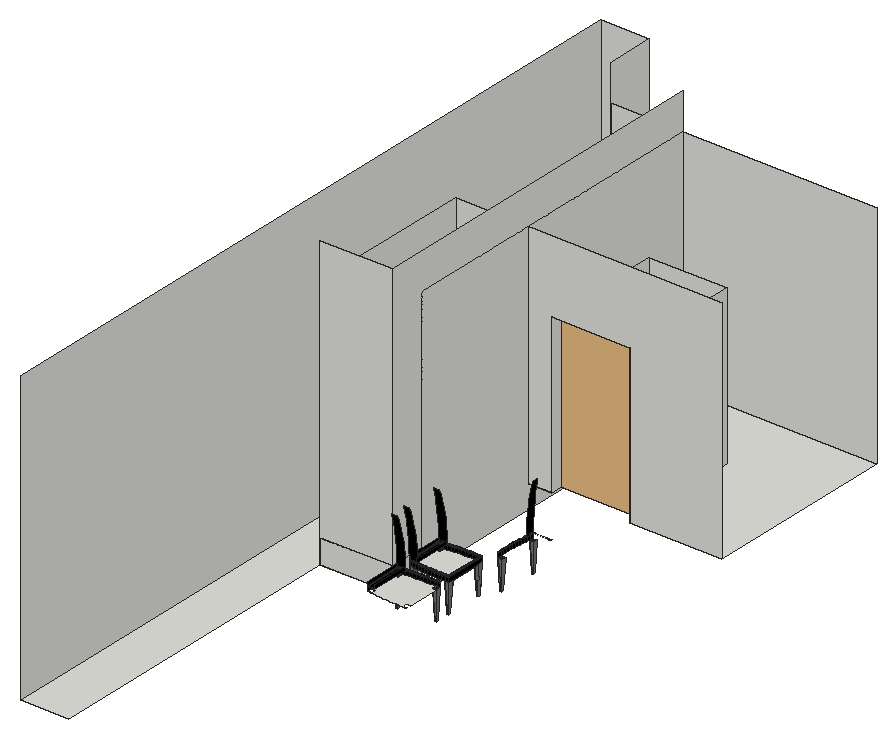
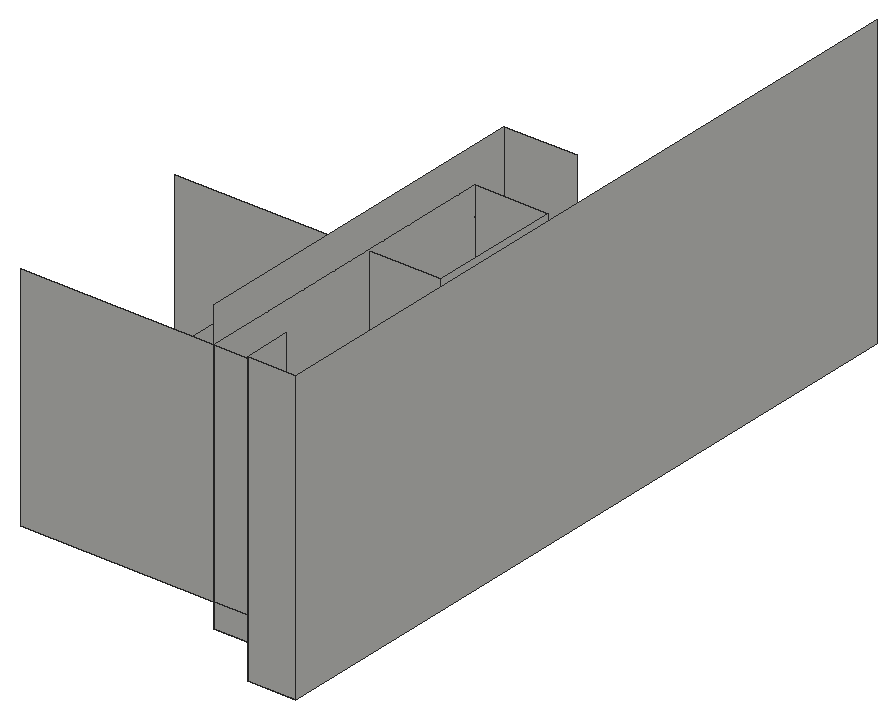
# SketchUp Ruby script. Lengths in inches.
U = 1.inch
M = Sketchup.active_model
def pt(a) = Geom::Point3d.new(a.map { |v| v * U })
def face(e, loops, mat)
  f = e.add_face(loops[0].map { |a| pt(a) })
  loops[1..].each { |l| e.add_face(l.map { |a| pt(a) }).erase! }
  f.material = f.back_material = mat if mat
  f
end
# faces: each face lists its corners as indices into pts; further lists are holes
def faces(e, pts, list, mat = nil) = list.each { |f| face(e, (f[0].is_a?(Array) ? f : [f]).map { |l| l.map { |i| pts[i] } }, mat) }
# xy, xz, yz: faces in a plane at the given z, y or x. An outline is a flat list of corners, or four numbers for a rectangle; further outlines are holes
def ring(l) = l.size == 4 ? [[l[0], l[1]], [l[2], l[1]], [l[2], l[3]], [l[0], l[3]]] : l.each_slice(2).to_a
def flat(e, list, mat, &to3) = list.each { |f| face(e, (f[0].is_a?(Array) ? f : [f]).map { |l| ring(l).map { |u, v| to3.(u, v) } }, mat) }
def xy(e, z, list, mat = nil) = flat(e, list, mat) { |x, y| [x, y, z] }
def xz(e, y, list, mat = nil) = flat(e, list, mat) { |x, z| [x, y, z] }
def yz(e, x, list, mat = nil) = flat(e, list, mat) { |y, z| [x, y, z] }
def lines(e, pts, list) = list.each { |a, b| e.add_line(pt(pts[a]), pt(pts[b])) }
# prism: a flat outline (further loops are holes) pulled along v
def prism(e, loops, v, mat = nil)
  f = face(e, loops, mat); d = Geom::Vector3d.new(v.map { |x| x * U })
  f.pushpull(f.normal.samedirection?(d) ? d.length : -d.length)
end
def box(e, o, s, mat = nil) = prism(e, [[o, [o[0] + s[0], o[1], o[2]], [o[0] + s[0], o[1] + s[1], o[2]], [o[0], o[1] + s[1], o[2]]]], [0, 0, s[2]], mat)
def at(x, y, z, deg = 0) = Geom::Transformation.translation(pt([x, y, z])) * Geom::Transformation.rotation(ORIGIN, Z_AXIS, deg.degrees)
def axes(o, x, y, z) = Geom::Transformation.new([*x, 0, *y, 0, *z, 0, *pt(o).to_a, 1])
def part(name) = M.definitions.add(name)
# library, detail: a bought-in or finely detailed component or shape, given as its bounding box
def library(name, o, s) = part(name).tap { |d| box(d.entities, o, s) }
def detail(e, o, s) = box(e.add_group.entities, o, s)
def put(e, d, t, mat = nil) = e.add_instance(d, t).tap { |i| i.material = mat if mat }
def group(e, t, mat = nil) = e.add_group.tap { |g| g.transformation = t; g.material = mat if mat }.entities
root = M.entities
M.materials.add("Color_008").color = [30, 30, 30]
M.materials.add("[Color M09]").color = [0, 0, 0]
M.materials.add("[Metal Seamed]").color = [118, 119, 115]
c1 = library("Group5\#2",[-22.22,-6.35,0],[42.52,9.29,84.25])
xy(root,0,[[0,0,24,360],[24,156,60,336]])
xy(root,12,[[24,156,60,174],[24,240,72,240,72,300,110.625,300,110.625,240,156,240,156,336,24,336]])
xy(root,12,[[81.769,130.997,82.586,131.814],[100.046,132.018,100.863,132.835],[100.046,139.647,100.863,140.464],[81.769,140.669,82.586,141.485],[81.769,156.903,82.586,157.72],
  [100.046,157.924,100.863,158.741],[104.815,166.733,105.632,167.55],[105.836,185.01,106.653,185.827]],"Color_008")
xy(root,26.704,[[96.409,112.95,94.702,112.965,92.996,113.008,91.291,113.079,89.587,113.178,87.885,113.306,86.185,113.462,84.488,113.646,82.795,113.858,81.105,114.098,83.25,114.098,83.25,116.244,81.105,116.244,81.105,130.333,83.25,130.333,83.25,132.478,81.105,132.478,82.795,132.718,84.488,132.931,86.185,133.115,87.885,133.271,89.587,133.398,91.291,133.498,92.996,133.569,94.702,133.612,96.409,133.626,98.115,133.612,99.822,133.57,101.527,133.499,99.382,133.499,99.382,131.354,101.527,131.354,101.527,115.223,99.382,115.223,99.382,113.077,101.527,113.077,99.822,113.007,98.115,112.964],[96.409,138.856,94.702,138.871,92.996,138.913,91.291,138.984,89.587,139.084,87.885,139.212,86.185,139.367,84.488,139.552,82.795,139.764,81.105,140.004,83.25,140.004,83.25,142.15,81.105,142.15,81.105,156.239,83.25,156.239,83.25,158.384,81.105,158.384,82.795,158.624,84.488,158.837,86.185,159.021,87.885,159.177,89.587,159.304,91.291,159.404,92.996,159.475,94.702,159.517,96.409,159.532,98.115,159.518,99.822,159.476,101.527,159.405,99.382,159.405,99.382,157.26,101.527,157.26,101.527,141.129,99.382,141.129,99.382,138.983,101.527,138.983,99.822,138.913,98.115,138.87]])
xy(root,26.704,[[81.105,130.333,83.25,132.478],[99.382,131.354,101.527,133.499],[99.382,138.983,101.527,141.129],[81.105,140.004,83.25,142.15],[81.105,156.239,83.25,158.384],
  [99.382,157.26,101.527,159.405],[104.151,166.069,106.296,168.214],[105.172,184.346,107.317,186.491]],"Color_008")
xy(root,28.845,[[81.105,114.098,84.642,132.478],[81.105,140.004,84.642,158.384]],"[Color M09]")
xz(root,132.478,[[81.105,28.845,84.642,28.845,84.773,30.816,84.825,32.79,84.797,34.764,84.689,36.736,84.502,38.701,84.235,40.658,83.89,42.602,83.466,44.53,82.965,46.44,82.387,48.328,81.733,50.191,81.004,52.027,78.554,52.027,78.952,50.121,79.316,48.208,79.647,46.29,79.945,44.365,80.208,42.436,80.438,40.503,80.634,38.566,80.797,36.626,80.925,34.683,81.019,32.738,81.079,30.792]],"[Color M09]")
xz(root,140.004,[[81.105,28.845,81.079,30.792,81.019,32.738,80.925,34.683,80.797,36.626,80.634,38.566,80.438,40.503,80.208,42.436,79.945,44.365,79.647,46.29,79.316,48.208,78.952,50.121,78.554,52.027,81.004,52.027,81.733,50.191,82.387,48.328,82.965,46.44,83.466,44.53,83.89,42.602,84.235,40.658,84.502,38.701,84.689,36.736,84.797,34.764,84.825,32.79,84.773,30.816,84.642,28.845]],"[Color M09]")
xz(root,156,[[24,0,60,12],[24,12,60,144]])
xz(root,158.384,[[81.105,28.845,84.642,28.845,84.773,30.816,84.825,32.79,84.797,34.764,84.689,36.736,84.502,38.701,84.235,40.658,83.89,42.602,83.466,44.53,82.965,46.44,82.387,48.328,81.733,50.191,81.004,52.027,78.554,52.027,78.952,50.121,79.316,48.208,79.647,46.29,79.945,44.365,80.208,42.436,80.438,40.503,80.634,38.566,80.797,36.626,80.925,34.683,81.019,32.738,81.079,30.792]],"[Color M09]")
xz(root,174,[[24,12,60,126]])
xz(root,240,[[24,12,72,12,72,90,110.625,90,110.625,12,156,12,156,126,24,126]])
xz(root,300,[[72,12,110.625,90]])
xz(root,336,[[24,0,60,12],[24,12,60,126],[60,12,156,126]])
xz(root,360,[[0,0,24,144]])
yz(root,0,[[0,0,360,144]])
yz(root,24,[[156,0,336,12],[336,0,360,144],[174,12,240,126]])
yz(root,60,[[156,0,336,0,336,126,174,126,174,12,156,12],[156,12,174,12,174,126,336,126,336,144,156,144]])
yz(root,72,[[240,12,300,90]])
yz(root,81.105,[[114.098,26.704,132.478,28.845],[140.004,26.704,158.384,28.845]],"[Color M09]")
yz(root,101.527,[[138.983,26.704,159.405,28.845]],"[Color M09]")
yz(root,105.172,[[182.954,28.845,186.491,28.845,186.517,30.792,186.577,32.738,186.671,34.683,186.799,36.626,186.962,38.566,187.158,40.503,187.388,42.436,187.651,44.365,187.949,46.29,188.28,48.208,188.644,50.121,189.042,52.027,186.592,52.027,185.863,50.191,185.209,48.328,184.631,46.44,184.13,44.53,183.706,42.602,183.361,40.658,183.094,38.701,182.907,36.736,182.799,34.764,182.771,32.79,182.823,30.816]],"[Color M09]")
yz(root,110.625,[[240,12,300,90]])
p = [[82.586,130.997,12],[83.25,130.333,26.704],[81.105,130.333,26.704],[81.769,130.997,12],[81.105,132.478,26.704],[81.769,131.814,12],
  [82.586,131.814,12],[83.25,132.478,26.704],[100.863,132.018,12],[101.527,131.354,26.704],[99.382,131.354,26.704],[100.046,132.018,12],
  [99.382,133.499,26.704],[100.046,132.835,12],[100.863,132.835,12],[101.527,133.499,26.704],[100.863,139.647,12],[101.527,138.983,26.704],
  [99.382,138.983,26.704],[100.046,139.647,12],[99.382,141.129,26.704],[100.046,140.464,12],[100.863,140.464,12],[101.527,141.129,26.704],
  [82.586,140.669,12],[83.25,140.004,26.704],[81.105,140.004,26.704],[81.769,140.669,12],[81.105,142.15,26.704],[81.769,141.485,12],
  [82.586,141.485,12],[83.25,142.15,26.704],[82.586,156.903,12],[83.25,156.239,26.704],[81.105,156.239,26.704],[81.769,156.903,12],
  [81.105,158.384,26.704],[81.769,157.72,12],[82.586,157.72,12],[83.25,158.384,26.704],[100.863,157.924,12],[101.527,157.26,26.704],
  [99.382,157.26,26.704],[100.046,157.924,12],[99.382,159.405,26.704],[100.046,158.741,12],[100.863,158.741,12],[101.527,159.405,26.704],
  [105.632,166.733,12],[106.296,166.069,26.704],[104.151,166.069,26.704],[104.815,166.733,12],[104.151,168.214,26.704],[104.815,167.55,12],
  [105.632,167.55,12],[106.296,168.214,26.704],[106.653,185.01,12],[107.317,184.346,26.704],[105.172,184.346,26.704],[105.836,185.01,12],
  [105.172,186.491,26.704],[105.836,185.827,12],[106.653,185.827,12],[107.317,186.491,26.704],[82.795,132.718,28.845],[82.795,132.718,26.704],
  [81.105,132.478,28.845],[84.488,132.931,28.845],[84.488,132.931,26.704],[86.185,133.115,28.845],[86.185,133.115,26.704],[87.885,133.271,28.845],
  [87.885,133.271,26.704],[89.587,133.398,28.845],[89.587,133.398,26.704],[91.291,133.498,28.845],[91.291,133.498,26.704],[92.996,133.569,28.845],
  [92.996,133.569,26.704],[99.822,133.57,28.845],[99.822,133.57,26.704],[101.527,133.499,28.845],[94.702,133.612,26.704],[94.702,133.612,28.845],
  [96.409,133.626,26.704],[96.409,133.626,28.845],[98.115,133.612,26.704],[98.115,133.612,28.845],[92.996,138.913,26.704],[92.996,138.913,28.845],
  [91.291,138.984,28.845],[91.291,138.984,26.704],[94.702,138.871,28.845],[94.702,138.871,26.704],[96.409,138.856,28.845],[96.409,138.856,26.704],
  [98.115,138.87,28.845],[98.115,138.87,26.704],[99.822,138.913,28.845],[99.822,138.913,26.704],[101.527,138.983,28.845],[89.587,139.084,28.845],
  [89.587,139.084,26.704],[87.885,139.212,28.845],[87.885,139.212,26.704],[86.185,139.367,28.845],[86.185,139.367,26.704],[84.488,139.552,28.845],
  [84.488,139.552,26.704],[82.795,139.764,28.845],[82.795,139.764,26.704],[81.105,140.004,28.845],[82.795,158.624,28.845],[82.795,158.624,26.704],
  [81.105,158.384,28.845],[84.488,158.837,28.845],[84.488,158.837,26.704],[86.185,159.021,28.845],[86.185,159.021,26.704],[87.885,159.177,28.845],
  [87.885,159.177,26.704],[89.587,159.304,28.845],[89.587,159.304,26.704],[91.291,159.404,28.845],[91.291,159.404,26.704],[92.996,159.475,28.845],
  [92.996,159.475,26.704],[99.822,159.476,28.845],[99.822,159.476,26.704],[101.527,159.405,28.845],[94.702,159.517,26.704],[94.702,159.517,28.845],
  [96.409,159.532,26.704],[96.409,159.532,28.845],[98.115,159.518,26.704],[98.115,159.518,28.845],[104.08,167.774,26.704],[104.08,167.774,28.845],
  [104.151,166.069,28.845],[104.038,169.481,26.704],[104.038,169.481,28.845],[104.024,171.1875,26.704],[104.024,171.1875,28.845],[104.038,172.894,26.704],
  [104.038,172.894,28.845],[104.081,174.6,26.704],[104.081,174.6,28.845],[104.152,176.305,28.845],[104.152,176.305,26.704],[104.252,178.009,28.845],
  [104.252,178.009,26.704],[104.379,179.711,28.845],[104.379,179.711,26.704],[104.535,181.411,28.845],[104.535,181.411,26.704],[104.719,183.108,28.845],
  [104.719,183.108,26.704],[104.932,184.801,28.845],[104.932,184.801,26.704],[105.172,186.491,28.845],[81.079,132.478,30.792],[81.079,114.098,30.792],
  [81.105,114.098,28.845],[81.115,132.47,28.992],[81.115,114.107,28.992],[84.773,132.478,30.816],[84.642,132.478,28.845],[84.642,114.098,28.845],
  [84.773,114.098,30.816],[82.796,132.709,28.992],[84.489,132.921,28.992],[86.186,133.105,28.992],[87.886,133.261,28.992],[89.587,133.389,28.992],
  [91.291,133.488,28.992],[92.996,133.559,28.992],[99.821,133.56,28.992],[101.517,133.49,28.992],[94.702,133.602,28.992],[96.409,133.616,28.992],
  [98.115,133.602,28.992],[92.996,138.923,28.992],[91.291,138.994,28.992],[94.702,138.88,28.992],[96.409,138.866,28.992],[98.115,138.88,28.992],
  [99.821,138.922,28.992],[101.517,138.992,28.992],[89.587,139.093,28.992],[101.517,159.396,28.992],[87.886,139.221,28.992],[86.186,139.377,28.992],
  [84.489,139.561,28.992],[82.796,139.773,28.992],[81.115,140.013,28.992],[81.079,158.384,30.792],[81.079,140.004,30.792],[81.115,158.376,28.992],
  [84.773,158.384,30.816],[84.642,158.384,28.845],[84.642,140.004,28.845],[84.773,140.004,30.816],[82.796,158.615,28.992],[84.489,158.827,28.992],
  [86.186,159.011,28.992],[87.886,159.167,28.992],[89.587,159.295,28.992],[91.291,159.394,28.992],[92.996,159.465,28.992],[99.821,159.466,28.992],
  [94.702,159.508,28.992],[96.409,159.522,28.992],[98.115,159.508,28.992],[104.09,167.775,28.992],[104.16,166.079,28.992],[104.048,169.481,28.992],
  [104.034,171.1875,28.992],[104.048,172.894,28.992],[104.091,174.6,28.992],[104.162,176.305,28.992],[104.261,178.009,28.992],[104.389,179.71,28.992],
  [104.545,181.41,28.992],[104.729,183.107,28.992],[104.941,184.8,28.992],[105.18,186.481,28.992],[81.143,132.445,29.137],[81.143,114.132,29.137],
  [81.143,123.288,29.137],[82.8,132.68,29.137],[84.493,132.893,29.137],[86.189,133.077,29.137],[87.888,133.233,29.137],[89.589,133.36,29.137],
  [91.292,133.46,29.137],[92.997,133.531,29.137],[94.703,133.573,29.137],[98.115,133.574,29.137],[99.82,133.531,29.137],[101.489,133.462,29.137],
  [96.409,133.588,29.137],[92.997,138.952,29.137],[91.292,139.023,29.137],[94.703,138.909,29.137],[96.409,138.895,29.137],[98.115,138.909,29.137],
  [99.82,138.951,29.137],[101.489,139.02,29.137],[89.589,139.122,29.137],[101.489,159.368,29.137],[87.888,139.25,29.137],[86.189,139.406,29.137],
  [84.493,139.59,29.137],[82.8,139.802,29.137],[81.143,140.038,29.137],[81.143,158.351,29.137],[81.143,149.194,29.137],[82.8,158.586,29.137],
  [84.493,158.798,29.137],[86.189,158.983,29.137],[87.888,159.138,29.137],[89.589,159.266,29.137],[91.292,159.365,29.137],[92.997,159.436,29.137],
  [94.703,159.479,29.137],[98.115,159.48,29.137],[99.82,159.437,29.137],[96.409,159.494,29.137],[104.119,167.776,29.137],[104.188,166.107,29.137],
  [104.076,169.481,29.137],[104.0625,171.1875,29.137],[104.077,172.893,29.137],[104.119,174.599,29.137],[104.191,176.304,29.137],[104.29,178.007,29.137],
  [104.417,179.708,29.137],[104.573,181.407,29.137],[104.757,183.103,29.137],[104.97,184.796,29.137],[105.205,186.453,29.137],[81.191,132.404,29.276],
  [81.191,123.288,29.276],[82.806,132.633,29.276],[84.498,132.846,29.276],[86.194,133.03,29.276],[87.892,133.185,29.276],[89.592,133.313,29.276],
  [91.295,133.412,29.276],[92.999,133.483,29.276],[92.998,133.483,29.276],[99.819,133.484,29.276],[101.441,133.417,29.276],[94.703,133.526,29.276],
  [96.409,133.54,29.276],[98.114,133.526,29.276],[92.999,138.999,29.276],[94.703,138.956,29.276],[96.409,138.942,29.276],[98.114,138.956,29.276],
  [99.819,138.998,29.276],[91.295,139.07,29.276],[89.592,139.169,29.276],[92.998,138.999,29.276],[101.441,139.065,29.276],[101.441,159.323,29.276],
  [87.892,139.297,29.276],[86.194,139.453,29.276],[84.498,139.637,29.276],[82.806,139.849,29.276],[81.191,140.079,29.276],[81.191,149.194,29.276],
  [81.191,158.31,29.276],[82.806,158.539,29.276],[84.498,158.751,29.276],[86.194,158.935,29.276],[87.892,159.091,29.276],[89.592,159.219,29.276],
  [91.295,159.318,29.276],[92.999,159.389,29.276],[92.998,159.389,29.276],[99.819,159.39,29.276],[94.703,159.432,29.276],[96.409,159.446,29.276],
  [98.114,159.432,29.276],[104.166,167.777,29.276],[104.233,166.155,29.276],[104.124,169.482,29.276],[104.11,171.1875,29.276],[104.124,172.893,29.276],
  [104.167,174.597,29.276],[104.167,174.598,29.276],[104.238,176.301,29.276],[104.337,178.004,29.276],[104.465,179.704,29.276],[104.62,181.402,29.276],
  [104.804,183.098,29.276],[105.017,184.79,29.276],[105.246,186.405,29.276],[114.362,186.405,29.276],[114.362,186.453,29.137],[81.256,132.347,29.408],
  [81.256,123.288,29.408],[82.815,132.569,29.408],[84.506,132.781,29.408],[86.2,132.965,29.408],[87.897,133.121,29.408],[89.597,133.248,29.408],
  [91.298,133.347,29.408],[93,133.418,29.408],[93.002,133.418,29.408],[94.705,133.461,29.408],[98.113,133.461,29.408],[99.817,133.419,29.408],
  [101.376,133.354,29.408],[96.409,133.475,29.408],[94.705,139.021,29.408],[96.409,139.007,29.408],[98.113,139.021,29.408],[93,139.064,29.408],
  [91.298,139.135,29.408],[93.002,139.064,29.408],[99.817,139.063,29.408],[101.376,139.128,29.408],[89.597,139.234,29.408],[101.376,159.26,29.408],
  [87.897,139.362,29.408],[86.2,139.517,29.408],[84.506,139.701,29.408],[82.815,139.913,29.408],[81.256,140.135,29.408],[81.256,149.194,29.408],
  [81.256,158.253,29.408],[82.815,158.475,29.408],[84.506,158.687,29.408],[86.2,158.871,29.408],[87.897,159.026,29.408],[89.597,159.154,29.408],
  [91.298,159.253,29.408],[93,159.324,29.408],[93.002,159.324,29.408],[94.705,159.367,29.408],[98.113,159.367,29.408],[99.817,159.325,29.408],
  [96.409,159.381,29.408],[104.231,167.779,29.408],[104.296,166.22,29.408],[104.189,169.483,29.408],[104.175,171.1875,29.408],[104.189,172.891,29.408],
  [104.232,174.594,29.408],[104.232,174.596,29.408],[104.303,176.298,29.408],[104.402,177.999,29.408],[104.529,179.699,29.408],[104.685,181.396,29.408],
  [104.869,183.09,29.408],[105.081,184.781,29.408],[105.303,186.34,29.408],[114.362,186.34,29.408],[81.338,132.276,29.531],[81.338,123.288,29.531],
  [82.826,132.488,29.531],[84.515,132.7,29.531],[86.208,132.883,29.531],[87.904,133.039,29.531],[89.602,133.166,29.531],[91.302,133.266,29.531],
  [93.002,133.336,29.531],[93.006,133.337,29.531],[94.706,133.379,29.531],[98.112,133.38,29.531],[99.814,133.337,29.531],[101.294,133.276,29.531],
  [96.409,133.393,29.531],[93.006,139.146,29.531],[94.706,139.103,29.531],[96.409,139.089,29.531],[98.112,139.103,29.531],[99.814,139.145,29.531],
  [91.302,139.217,29.531],[89.602,139.316,29.531],[93.002,139.146,29.531],[101.294,139.206,29.531],[101.294,159.182,29.531],[87.904,139.443,29.531],
  [86.208,139.599,29.531],[84.515,139.783,29.531],[82.826,139.994,29.531],[81.338,140.206,29.531],[81.338,149.194,29.531],[81.338,158.182,29.531],
  [82.826,158.394,29.531],[84.515,158.606,29.531],[86.208,158.789,29.531],[87.904,158.945,29.531],[89.602,159.072,29.531],[91.302,159.171,29.531],
  [93.002,159.242,29.531],[93.006,159.242,29.531],[94.706,159.285,29.531],[98.112,159.285,29.531],[99.814,159.243,29.531],[96.409,159.299,29.531],
  [104.313,167.782,29.531],[104.374,166.302,29.531],[104.27,169.484,29.531],[104.257,171.1875,29.531],[104.271,172.89,29.531],[104.313,174.591,29.531],
  [104.314,174.594,29.531],[104.384,176.294,29.531],[104.484,177.994,29.531],[104.611,179.692,29.531],[104.767,181.388,29.531],[104.95,183.081,29.531],
  [105.162,184.77,29.531],[105.374,186.258,29.531],[114.362,186.258,29.531],[93.004,139.243,29.641],[91.307,139.314,29.641],[93.01,139.243,29.641],
  [94.708,139.2,29.641],[96.409,139.186,29.641],[98.11,139.2,29.641],[99.811,139.242,29.641],[101.197,139.299,29.641],[89.609,139.413,29.641],
  [101.197,159.089,29.641],[87.912,139.54,29.641],[86.218,139.695,29.641],[84.527,139.879,29.641],[82.839,140.091,29.641],[81.435,140.29,29.641],
  [81.435,149.194,29.641],[81.435,158.098,29.641],[82.839,158.298,29.641],[84.527,158.509,29.641],[86.218,158.693,29.641],[87.912,158.848,29.641],
  [89.609,158.975,29.641],[91.307,159.075,29.641],[93.004,159.145,29.641],[93.01,159.145,29.641],[94.708,159.188,29.641],[98.11,159.188,29.641],
  [99.811,159.146,29.641],[96.409,159.202,29.641]]
faces(root,p,[[0,1,2,3],[3,2,4,5],[1,0,6,7],[8,9,10,11],[11,10,12,13],[9,8,14,15],[7,6,5,4],[15,14,13,12],
  [16,17,18,19],[20,21,19,18],[22,23,17,16],[24,25,26,27],[28,29,27,26],[30,31,25,24],[23,22,21,20],[31,30,29,28],
  [32,33,34,35],[35,34,36,37],[33,32,38,39],[40,41,42,43],[43,42,44,45],[41,40,46,47],[39,38,37,36],[47,46,45,44],
  [48,49,50,51],[51,50,52,53],[49,48,54,55],[55,54,53,52],[56,57,58,59],[59,58,60,61],[57,56,62,63],[63,62,61,60]],"[Metal Seamed]")
faces(root,p,[[64,65,4,66],[67,68,65,64],[69,70,68,67],[71,72,70,69],[73,74,72,71],[75,76,74,73],[77,78,76,75],[79,80,15,81],
  [77,78,82,83],[83,82,84,85],[85,84,86,87],[87,86,80,79],[88,89,90,91],[88,89,92,93],[93,92,94,95],[95,94,96,97],
  [97,96,98,99],[99,98,100,17],[91,90,101,102],[102,101,103,104],[104,103,105,106],[106,105,107,108],[108,107,109,110],[110,109,111,26],
  [112,113,36,114],[115,116,113,112],[117,118,116,115],[119,120,118,117],[121,122,120,119],[123,124,122,121],[125,126,124,123],[127,128,47,129],
  [125,126,130,131],[131,130,132,133],[133,132,134,135],[135,134,128,127],[136,137,138,50],[139,140,137,136],[141,142,140,139],[143,144,142,141],
  [145,146,144,143],[145,146,147,148],[148,147,149,150],[150,149,151,152],[152,151,153,154],[154,153,155,156],[156,155,157,158],[158,157,159,60],
  [66,160,161,162],[163,66,162,164],[165,166,167,168],[169,64,66,163],[170,67,64,169],[171,69,67,170],[172,71,69,171],[173,73,71,172],
  [174,75,73,173],[175,77,75,174],[176,79,81,177],[175,77,83,178],[178,83,85,179],[179,85,87,180],[180,87,79,176],[89,181,182,90],
  [89,181,183,92],[92,183,184,94],[94,184,185,96],[96,185,186,98],[98,186,187,100],[90,182,188,101],[189,129,100,187],[101,188,190,103],
  [103,190,191,105],[105,191,192,107],[107,192,193,109],[109,193,194,111],[114,195,196,111],[197,114,111,194],[198,199,200,201],[202,112,114,197],
  [203,115,112,202],[204,117,115,203],[205,119,117,204],[206,121,119,205],[207,123,121,206],[208,125,123,207],[209,127,129,189],[208,125,131,210],
  [210,131,133,211],[211,133,135,212],[212,135,127,209],[137,213,214,138],[140,215,213,137],[142,216,215,140],[144,217,216,142],[146,218,217,144],
  [146,218,219,147],[147,219,220,149],[149,220,221,151],[151,221,222,153],[153,222,223,155],[155,223,224,157],[157,224,225,159],[226,163,164,227,228],
  [229,169,163,226],[230,170,169,229],[231,171,170,230],[232,172,171,231],[233,173,172,232],[234,174,173,233],[175,174,234,235],[235,175,178,236],
  [237,180,176,238],[238,176,177,239],[236,178,179,240],[240,179,180,237],[182,181,241,242],[181,241,243,183],[183,243,244,184],[184,244,245,185],
  [185,245,246,186],[186,246,247,187],[182,242,248,188],[249,189,187,247],[188,248,250,190],[190,250,251,191],[191,251,252,192],[192,252,253,193],
  [193,253,254,194],[255,197,194,254,256],[257,202,197,255],[258,203,202,257],[259,204,203,258],[260,205,204,259],[261,206,205,260],[262,207,206,261],
  [208,207,262,263],[263,208,210,264],[265,212,209,266],[266,209,189,249],[264,210,211,267],[267,211,212,265],[213,268,269,214],[215,270,268,213],
  [216,271,270,215],[217,272,271,216],[218,273,272,217],[219,218,273,274],[219,274,275,220],[220,275,276,221],[221,276,277,222],[222,277,278,223],
  [223,278,279,224],[224,279,280,225],[281,226,228,282],[283,229,226,281],[284,230,229,283],[285,231,230,284],[286,232,231,285],[287,233,232,286],
  [288,234,233,287],[289,235,234,288,290],[291,238,239,292],[235,236,293,289],[293,236,240,294],[294,240,237,295],[295,237,238,291],[243,241,296,297],
  [243,297,298,244],[244,298,299,245],[245,299,300,246],[242,301,302,248],[241,296,303,301,242],[246,300,304,247],[305,249,247,304],[248,302,306,250],
  [250,306,307,251],[251,307,308,252],[252,308,309,253],[253,309,310,254],[254,310,311,256],[312,255,256,311],[313,257,255,312],[314,258,257,313],
  [315,259,258,314],[316,260,259,315],[317,261,260,316],[318,262,261,317],[319,263,262,318,320],[321,266,249,305],[263,264,322,319],[322,264,267,323],
  [323,267,265,324],[324,265,266,321],[268,325,326,269],[270,327,325,268],[271,328,327,270],[272,329,328,271],[272,273,330,329],[273,330,331,332,274],
  [274,332,333,275],[275,333,334,276],[276,334,335,277],[277,335,336,278],[278,336,337,279],[279,337,338,280],[280,338,339,340],[341,281,282,342],
  [343,283,281,341],[344,284,283,343],[345,285,284,344],[346,286,285,345],[347,287,286,346],[348,288,287,347],[290,288,348,349],[349,350,289,290],
  [289,293,351,350],[352,295,291,353],[353,291,292,354],[351,293,294,355],[355,294,295,352],[297,356,357,298],[298,357,358,299],[301,303,359,360],
  [297,296,361,356],[359,361,296,303],[299,358,362,300],[300,362,363,304],[301,360,364,302],[365,305,304,363],[302,364,366,306],[306,366,367,307],
  [307,367,368,308],[308,368,369,309],[309,369,370,310],[310,370,371,311],[372,312,311,371],[373,313,312,372],[374,314,313,373],[375,315,314,374],
  [376,316,315,375],[377,317,316,376],[378,318,317,377],[320,318,378,379],[379,380,319,320],[319,322,381,380],[382,324,321,383],[383,321,305,365],
  [381,322,323,384],[384,323,324,382],[325,385,386,326],[327,387,385,325],[328,388,387,327],[329,389,388,328],[329,330,390,389],[391,390,330,331],
  [332,331,391,392],[332,392,393,333],[333,393,394,334],[334,394,395,335],[335,395,396,336],[336,396,397,337],[337,397,398,338],[338,398,399,339],
  [400,341,342,401],[402,343,341,400],[403,344,343,402],[404,345,344,403],[405,346,345,404],[406,347,346,405],[407,348,347,406],[349,348,407,408],
  [409,408,349,350],[350,351,410,409],[411,352,353,412],[412,353,354,413],[410,351,355,414],[414,355,352,411],[356,361,415,416],[356,416,417,357],
  [357,417,418,358],[358,418,419,362],[360,420,421,364],[360,359,422,420],[415,422,359,361],[362,419,423,363],[424,365,363,423],[364,421,425,366],
  [366,425,426,367],[367,426,427,368],[368,427,428,369],[369,428,429,370],[370,429,430,371],[431,372,371,430],[432,373,372,431],[433,374,373,432],
  [434,375,374,433],[435,376,375,434],[436,377,376,435],[437,378,377,436],[379,378,437,438],[439,438,379,380],[380,381,440,439],[441,382,383,442],
  [442,383,365,424],[440,381,384,443],[443,384,382,441],[385,444,445,386],[387,446,444,385],[388,447,446,387],[389,448,447,388],[389,390,449,448],
  [449,450,391,390],[392,391,450,451],[392,451,452,393],[393,452,453,394],[394,453,454,395],[395,454,455,396],[396,455,456,397],[397,456,457,398],
  [398,457,458,399],[420,422,459,460],[416,415,461,462],[459,461,415,422],[416,462,463,417],[417,463,464,418],[418,464,465,419],[419,465,466,423],
  [420,460,467,421],[468,424,423,466],[421,467,469,425],[425,469,470,426],[426,470,471,427],[427,471,472,428],[428,472,473,429],[429,473,474,430],
  [475,431,430,474],[476,432,431,475],[477,433,432,476],[478,434,433,477],[479,435,434,478],[480,436,435,479],[481,437,436,480],[438,437,481,482],
  [482,483,439,438],[439,440,484,483],[485,441,442,486],[486,442,424,468],[484,440,443,487],[487,443,441,485]],"[Color M09]")
put(root,c1,axes([92.39,251.1,12],[0.9177,0,0],[0,0.9177,0],[0,0,0.9177]))
